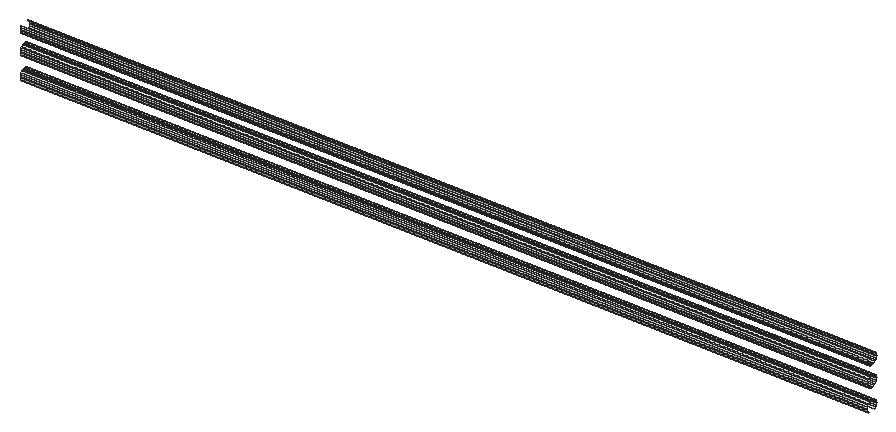
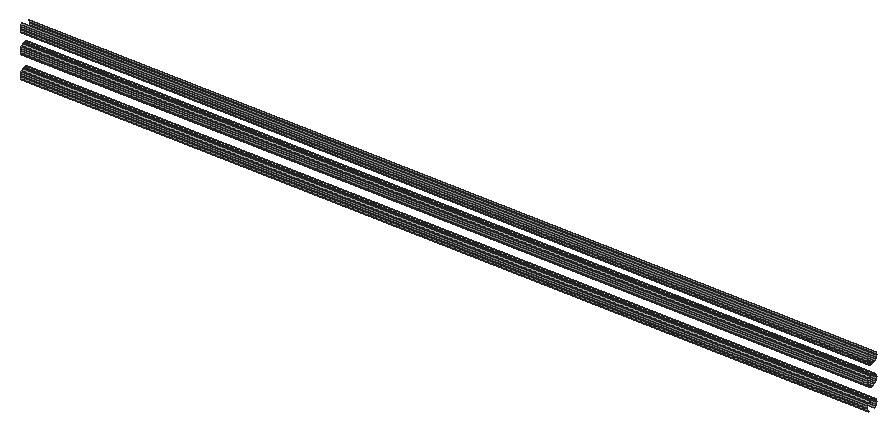
# SketchUp Ruby script. Lengths in inches.
U = 1.inch
M = Sketchup.active_model
def pt(a) = Geom::Point3d.new(a.map { |v| v * U })
def face(e, loops, mat)
  f = e.add_face(loops[0].map { |a| pt(a) })
  loops[1..].each { |l| e.add_face(l.map { |a| pt(a) }).erase! }
  f.material = f.back_material = mat if mat
  f
end
# faces: each face lists its corners as indices into pts; further lists are holes
def faces(e, pts, list, mat = nil) = list.each { |f| face(e, (f[0].is_a?(Array) ? f : [f]).map { |l| l.map { |i| pts[i] } }, mat) }
# xy, xz, yz: faces in a plane at the given z, y or x. An outline is a flat list of corners, or four numbers for a rectangle; further outlines are holes
def ring(l) = l.size == 4 ? [[l[0], l[1]], [l[2], l[1]], [l[2], l[3]], [l[0], l[3]]] : l.each_slice(2).to_a
def flat(e, list, mat, &to3) = list.each { |f| face(e, (f[0].is_a?(Array) ? f : [f]).map { |l| ring(l).map { |u, v| to3.(u, v) } }, mat) }
def xy(e, z, list, mat = nil) = flat(e, list, mat) { |x, y| [x, y, z] }
def xz(e, y, list, mat = nil) = flat(e, list, mat) { |x, z| [x, y, z] }
def yz(e, x, list, mat = nil) = flat(e, list, mat) { |y, z| [x, y, z] }
def lines(e, pts, list) = list.each { |a, b| e.add_line(pt(pts[a]), pt(pts[b])) }
# prism: a flat outline (further loops are holes) pulled along v
def prism(e, loops, v, mat = nil)
  f = face(e, loops, mat); d = Geom::Vector3d.new(v.map { |x| x * U })
  f.pushpull(f.normal.samedirection?(d) ? d.length : -d.length)
end
def box(e, o, s, mat = nil) = prism(e, [[o, [o[0] + s[0], o[1], o[2]], [o[0] + s[0], o[1] + s[1], o[2]], [o[0], o[1] + s[1], o[2]]]], [0, 0, s[2]], mat)
def at(x, y, z, deg = 0) = Geom::Transformation.translation(pt([x, y, z])) * Geom::Transformation.rotation(ORIGIN, Z_AXIS, deg.degrees)
def axes(o, x, y, z) = Geom::Transformation.new([*x, 0, *y, 0, *z, 0, *pt(o).to_a, 1])
def part(name) = M.definitions.add(name)
# library, detail: a bought-in or finely detailed component or shape, given as its bounding box
def library(name, o, s) = part(name).tap { |d| box(d.entities, o, s) }
def detail(e, o, s) = box(e.add_group.entities, o, s)
def put(e, d, t, mat = nil) = e.add_instance(d, t).tap { |i| i.material = mat if mat }
def group(e, t, mat = nil) = e.add_group.tap { |g| g.transformation = t; g.material = mat if mat }.entities
root = M.entities
M.materials.add("[Polished Concrete Old]").color = [229, 229, 229]
p = [[922.51,234.99,24.62],[922.51,234.6,25.125],[562.43,234.6,25.125],[562.43,234.99,24.62],[922.51,238.83,25.125],[922.51,238.4375,24.62],
  [562.43,238.4375,24.62],[562.43,238.83,25.125],[922.51,234.36,25.71],[562.43,234.36,25.71],[922.51,239.07,25.71],[562.43,239.07,25.71],
  [922.51,234.28,26.34],[562.43,234.28,26.34],[922.51,239.15,26.34],[562.43,239.15,26.34],[922.51,234.36,26.97],[562.43,234.36,26.97],
  [922.51,239.07,26.97],[562.43,239.07,26.97],[922.51,234.6,27.5625],[562.43,234.6,27.5625],[922.51,238.83,27.5625],[562.43,238.83,27.5625],
  [922.51,234.99,28.07],[562.43,234.99,28.07],[922.51,238.4375,28.07],[562.43,238.4375,28.07],[922.51,235.5,28.45],[562.43,235.5,28.45],
  [922.51,237.93,28.45],[562.43,237.93,28.45],[922.51,236.08,28.7],[562.43,236.08,28.7],[922.51,237.35,28.7],[562.43,237.35,28.7],
  [922.51,236.71,28.78],[562.43,236.71,28.78],[922.51,236.71,33.4],[922.51,236.08,33.49],[562.43,236.08,33.49],[562.43,236.71,33.4],
  [922.51,237.35,33.49],[562.43,237.35,33.49],[922.51,235.5,33.73],[562.43,235.5,33.73],[922.51,237.93,33.73],[562.43,237.93,33.73],
  [922.51,234.99,34.12],[562.43,234.99,34.12],[922.51,238.4375,34.12],[562.43,238.4375,34.12],[922.51,234.6,34.625],[562.43,234.6,34.625],
  [922.51,238.83,34.625],[562.43,238.83,34.625],[922.51,234.36,35.21],[562.43,234.36,35.21],[922.51,239.07,35.21],[562.43,239.07,35.21],
  [922.51,234.28,35.84],[562.43,234.28,35.84],[922.51,239.15,35.84],[562.43,239.15,35.84],[922.51,234.36,36.47],[562.43,234.36,36.47],
  [922.51,239.07,36.47],[562.43,239.07,36.47],[922.51,234.6,37.0625],[562.43,234.6,37.0625],[922.51,238.83,37.0625],[562.43,238.83,37.0625],
  [922.51,234.99,37.57],[562.43,234.99,37.57],[922.51,238.4375,37.57],[562.43,238.4375,37.57],[922.51,235.5,37.95],[562.43,235.5,37.95],
  [922.51,237.93,37.95],[562.43,237.93,37.95],[922.51,236.08,38.2],[562.43,236.08,38.2],[922.51,237.35,38.2],[562.43,237.35,38.2],
  [922.51,236.71,38.28],[562.43,236.71,38.28],[922.51,236.71,41.84],[922.51,236.08,41.93],[562.43,236.08,41.93],[562.43,236.71,41.84],
  [922.51,237.35,41.93],[562.43,237.35,41.93],[922.51,235.5,42.17],[562.43,235.5,42.17],[922.51,237.93,42.17],[562.43,237.93,42.17],
  [922.51,234.99,42.56],[562.43,234.99,42.56],[922.51,238.4375,42.56],[562.43,238.4375,42.56],[922.51,234.6,43.0625],[562.43,234.6,43.0625],
  [922.51,238.83,43.0625],[562.43,238.83,43.0625],[922.51,234.36,43.65],[562.43,234.36,43.65],[922.51,239.07,43.65],[562.43,239.07,43.65],
  [922.51,234.28,44.28],[562.43,234.28,44.28],[922.51,239.15,44.28],[562.43,239.15,44.28],[922.51,234.36,44.91],[562.43,234.36,44.91],
  [922.51,239.07,44.91],[562.43,239.07,44.91],[922.51,234.6,45.5],[562.43,234.6,45.5],[922.51,238.83,45.5],[562.43,238.83,45.5],
  [922.51,238.4375,46],[562.43,238.4375,46]]
faces(root,p,[[0,1,2,3],[4,5,6,7],[1,8,9,2],[10,4,7,11],[8,12,13,9],[14,10,11,15],[12,16,17,13],[18,14,15,19],
  [16,20,21,17],[22,18,19,23],[20,24,25,21],[26,22,23,27],[24,28,29,25],[30,26,27,31],[28,32,33,29],[34,30,31,35],
  [32,36,37,33],[36,34,35,37],[38,39,40,41],[42,38,41,43],[39,44,45,40],[46,42,43,47],[44,48,49,45],[50,46,47,51],
  [48,52,53,49],[54,50,51,55],[52,56,57,53],[58,54,55,59],[56,60,61,57],[62,58,59,63],[60,64,65,61],[66,62,63,67],
  [64,68,69,65],[70,66,67,71],[68,72,73,69],[74,70,71,75],[72,76,77,73],[78,74,75,79],[76,80,81,77],[82,78,79,83],
  [80,84,85,81],[84,82,83,85],[86,87,88,89],[90,86,89,91],[87,92,93,88],[94,90,91,95],[92,96,97,93],[98,94,95,99],
  [96,100,101,97],[102,98,99,103],[100,104,105,101],[106,102,103,107],[104,108,109,105],[110,106,107,111],[108,112,113,109],[114,110,111,115],
  [112,116,117,113],[118,114,115,119],[120,118,119,121]],"[Polished Concrete Old]")
